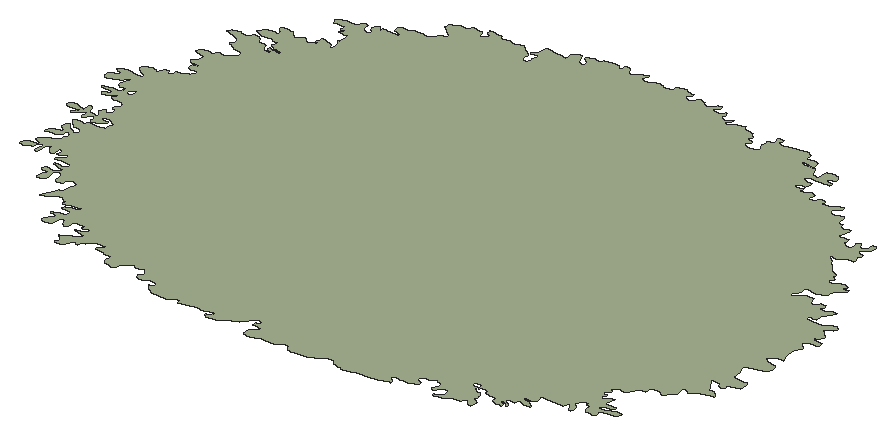
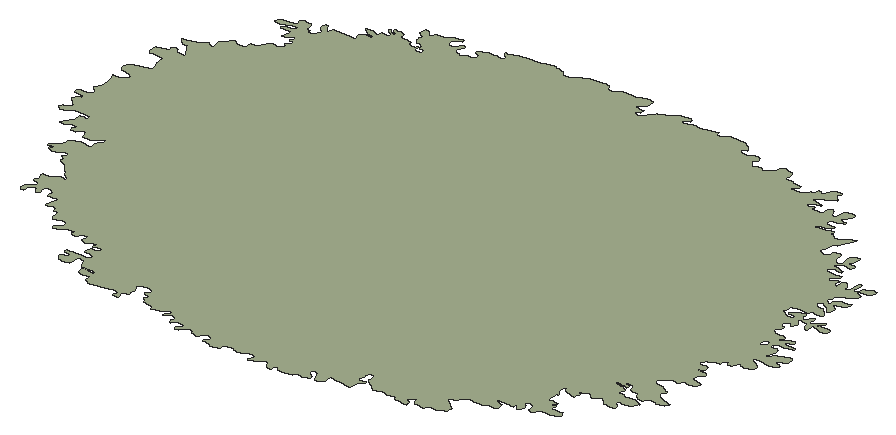
# SketchUp Ruby script. Lengths in inches.
U = 1.inch
M = Sketchup.active_model
def pt(a) = Geom::Point3d.new(a.map { |v| v * U })
def face(e, loops, mat)
  f = e.add_face(loops[0].map { |a| pt(a) })
  loops[1..].each { |l| e.add_face(l.map { |a| pt(a) }).erase! }
  f.material = f.back_material = mat if mat
  f
end
# faces: each face lists its corners as indices into pts; further lists are holes
def faces(e, pts, list, mat = nil) = list.each { |f| face(e, (f[0].is_a?(Array) ? f : [f]).map { |l| l.map { |i| pts[i] } }, mat) }
# xy, xz, yz: faces in a plane at the given z, y or x. An outline is a flat list of corners, or four numbers for a rectangle; further outlines are holes
def ring(l) = l.size == 4 ? [[l[0], l[1]], [l[2], l[1]], [l[2], l[3]], [l[0], l[3]]] : l.each_slice(2).to_a
def flat(e, list, mat, &to3) = list.each { |f| face(e, (f[0].is_a?(Array) ? f : [f]).map { |l| ring(l).map { |u, v| to3.(u, v) } }, mat) }
def xy(e, z, list, mat = nil) = flat(e, list, mat) { |x, y| [x, y, z] }
def xz(e, y, list, mat = nil) = flat(e, list, mat) { |x, z| [x, y, z] }
def yz(e, x, list, mat = nil) = flat(e, list, mat) { |y, z| [x, y, z] }
def lines(e, pts, list) = list.each { |a, b| e.add_line(pt(pts[a]), pt(pts[b])) }
# prism: a flat outline (further loops are holes) pulled along v
def prism(e, loops, v, mat = nil)
  f = face(e, loops, mat); d = Geom::Vector3d.new(v.map { |x| x * U })
  f.pushpull(f.normal.samedirection?(d) ? d.length : -d.length)
end
def box(e, o, s, mat = nil) = prism(e, [[o, [o[0] + s[0], o[1], o[2]], [o[0] + s[0], o[1] + s[1], o[2]], [o[0], o[1] + s[1], o[2]]]], [0, 0, s[2]], mat)
def at(x, y, z, deg = 0) = Geom::Transformation.translation(pt([x, y, z])) * Geom::Transformation.rotation(ORIGIN, Z_AXIS, deg.degrees)
def axes(o, x, y, z) = Geom::Transformation.new([*x, 0, *y, 0, *z, 0, *pt(o).to_a, 1])
def part(name) = M.definitions.add(name)
# library, detail: a bought-in or finely detailed component or shape, given as its bounding box
def library(name, o, s) = part(name).tap { |d| box(d.entities, o, s) }
def detail(e, o, s) = box(e.add_group.entities, o, s)
def put(e, d, t, mat = nil) = e.add_instance(d, t).tap { |i| i.material = mat if mat }
def group(e, t, mat = nil) = e.add_group.tap { |g| g.transformation = t; g.material = mat if mat }.entities
root = M.entities
M.materials.add("Boxwoodplan").color = [166, 177, 144]
xy(root,9.058,[[[229.854,67.129,229.743,67.133,229.648,67.159,229.592,67.215,229.591,67.317,229.617,67.382,229.68,67.445,229.729,67.509,229.788,67.606,229.601,67.635,229.511,67.644,229.531,67.732,229.617,67.79,229.648,67.8,229.643,67.846,229.554,67.877,229.438,67.837,229.341,67.706,229.199,67.551,229.038,67.464,228.932,67.441,228.872,67.416,228.856,67.373,228.711,67.281,228.518,67.251,228.429,67.26,228.348,67.306,228.348,67.328,228.394,67.359,228.484,67.437,228.553,67.483,228.463,67.498,228.351,67.48,228.231,67.436,228.037,67.454,227.94,67.447,227.814,67.403,227.613,67.356,227.524,67.349,227.486,67.443,227.478,67.465,227.411,67.473,227.322,67.454,227.154,67.336,226.954,67.328,226.724,67.353,226.557,67.446,226.415,67.61,226.598,67.702,226.499,67.756,226.363,67.772,226.237,67.749,226.164,67.697,226.084,67.672,225.968,67.738,225.926,67.806,226.013,67.847,226.04,67.907,226.045,67.957,226.004,68.009,225.931,68.085,225.846,68.117,225.759,68.064,225.692,68.038,225.636,68.08,225.62,68.103,225.596,68.121,225.566,68.111,225.487,68.058,225.415,68.01,225.339,67.923,225.328,67.79,225.256,67.749,225.206,67.723,225.146,67.725,225.047,67.746,224.961,67.793,224.917,67.861,224.908,67.951,224.917,68.018,224.93,68.04,224.911,68.08,224.698,68.1,224.766,68.135,224.739,68.136,224.647,68.13,224.477,68.146,224.4,68.173,224.383,68.206,224.397,68.224,224.523,68.314,224.52,68.371,224.436,68.393,224.276,68.39,224.146,68.319,224.048,68.233,223.974,68.199,223.926,68.172,223.925,68.154,223.962,68.101,223.946,68.046,223.875,68.081,223.812,68.121,223.751,68.072,223.728,68.017,223.697,67.904,223.649,67.855,223.576,67.822,223.485,67.816,223.415,67.841,223.397,67.874,223.404,67.892,223.425,67.932,223.447,67.991,223.416,68.048,223.315,68.149,223.429,68.229,223.49,68.269,223.569,68.285,223.637,68.315,223.692,68.37,223.776,68.476,223.705,68.503,223.625,68.511,223.493,68.53,223.454,68.565,223.462,68.584,223.536,68.62,223.698,68.657,223.741,68.709,223.736,68.748,223.71,68.764,223.56,68.711,223.514,68.732,223.515,68.752,223.537,68.814,223.376,68.825,223.296,68.833,223.242,68.826,223.234,68.806,223.218,68.71,223.203,68.642,223.162,68.591,223.115,68.578,223.095,68.594,223.036,68.639,222.992,68.757,222.952,68.783,222.925,68.784,222.872,68.777,222.865,68.757,222.863,68.641,222.808,68.523,222.748,68.449,222.668,68.419,222.589,68.422,222.542,68.448,222.509,68.506,222.51,68.564,222.563,68.677,222.677,68.784,222.698,68.803,222.684,68.823,222.658,68.829,222.577,68.847,222.497,68.86,222.47,68.875,222.476,68.895,222.497,68.914,222.645,68.982,222.807,69.005,222.849,69.108,222.823,69.169,222.776,69.191,222.748,69.187,222.585,69.168,222.545,69.2,222.551,69.22,222.579,69.279,222.736,69.334,222.908,69.403,222.957,69.442,222.943,69.463,222.847,69.436,222.675,69.417,222.531,69.372,222.442,69.386,222.415,69.392,222.422,69.412,222.442,69.426,222.497,69.47,222.47,69.507,222.442,69.503,222.36,69.511,222.305,69.56,222.291,69.601,222.263,69.597,222.181,69.575,222.024,69.489,221.874,69.413,221.8,69.38,221.745,69.392,221.758,69.412,221.778,69.452,221.804,69.469,221.829,69.55,221.878,69.65,221.91,69.759,221.961,69.812,222.035,69.852,222.079,69.972,222.101,70.112,222.12,70.227,222.116,70.285,222.071,70.321,221.991,70.335,221.904,70.335,221.831,70.31,221.821,70.245,221.821,70.184,221.788,70.124,221.7,70.087,221.644,70.096,221.605,70.155,221.595,70.216,221.569,70.337,221.563,70.4,221.523,70.453,221.495,70.475,221.458,70.491,221.399,70.479,221.364,70.46,221.363,70.428,221.355,70.366,221.357,70.229,221.382,70.167,221.374,70.103,221.324,70.038,221.275,70.01,221.237,69.998,221.2,70.003,221.158,70.011,221.14,70.039,221.136,70.166,221.157,70.223,221.202,70.276,221.218,70.306,221.209,70.334,221.152,70.34,221.071,70.346,221.033,70.362,221.01,70.39,221.007,70.453,221.023,70.483,221.057,70.499,221.23,70.472,221.308,70.497,221.358,70.526,221.418,70.573,221.432,70.636,221.409,70.662,221.365,70.664,221.287,70.67,221.195,70.681,221.094,70.717,221.076,70.746,221.081,70.76,221.101,70.763,221.16,70.775,221.336,70.761,221.425,70.787,221.438,70.844,221.412,70.907,221.34,70.946,221.261,70.953,221.147,70.946,221.048,70.921,220.964,70.939,220.96,70.968,220.981,70.997,221.027,71.054,221.094,71.11,221.147,71.19,221.138,71.224,221.094,71.241,221.029,71.24,220.911,71.14,220.871,71.141,220.837,71.161,220.858,71.22,220.875,71.287,220.831,71.35,220.791,71.366,220.771,71.367,220.766,71.352,220.77,71.306,220.767,71.164,220.726,71.102,220.686,71.108,220.652,71.131,220.554,71.262,220.529,71.327,220.505,71.355,220.489,71.344,220.434,71.293,220.399,71.234,220.418,71.103,220.423,71.037,220.403,70.971,220.354,70.962,220.319,70.978,220.309,71.023,220.329,71.155,220.339,71.233,220.339,71.27,220.324,71.282,220.309,71.272,220.229,71.237,220.19,71.183,220.18,71.12,220.141,71.077,220.004,70.987,219.965,70.977,219.92,70.986,219.841,71.026,219.82,71.056,219.824,71.089,219.857,71.151,219.955,71.237,220.044,71.263,220.134,71.263,220.229,71.267,220.169,71.318,220.017,71.404,220.001,71.466,220.054,71.503,220.145,71.573,220.264,71.635,220.383,71.709,220.418,71.723,220.444,71.746,220.471,71.789,220.474,71.882,220.506,72.003,220.507,72.065,220.486,72.086,220.465,72.095,220.402,72.109,220.368,72.104,220.365,72.088,220.376,71.996,220.335,71.934,220.287,71.899,220.209,71.871,220.138,71.858,219.978,71.833,219.943,71.839,219.929,71.853,219.93,71.86,219.938,71.901,219.955,71.947,219.997,71.995,220.067,72.042,220.125,72.063,220.184,72.065,220.222,72.068,220.242,72.075,220.265,72.096,220.261,72.121,220.206,72.151,220.138,72.207,220.106,72.264,220.102,72.331,220.115,72.382,220.168,72.426,220.194,72.432,220.205,72.425,220.224,72.411,220.267,72.35,220.316,72.304,220.445,72.226,220.518,72.192,220.554,72.177,220.574,72.184,220.598,72.206,220.604,72.222,220.616,72.263,220.6,72.32,220.558,72.366,220.525,72.389,220.492,72.401,220.432,72.401,220.358,72.404,220.314,72.446,220.228,72.519,220.17,72.569,220.131,72.617,220.131,72.646,220.155,72.671,220.212,72.698,220.247,72.703,220.288,72.7,220.348,72.679,220.409,72.677,220.445,72.684,220.48,72.726,220.528,72.757,220.588,72.764,220.659,72.764,220.8125,72.771,220.953,72.792,220.985,72.808,220.986,72.826,220.98,72.868,220.969,72.913,220.98,72.957,221.01,73.06,220.996,73.083,220.974,73.097,220.917,73.126,220.863,73.164,220.791,73.192,220.718,73.195,220.667,73.184,220.646,73.17,220.621,73.119,220.626,73.098,220.638,73.093,220.661,73.088,220.812,73.076,220.838,73.071,220.844,73.0625,220.834,73.046,220.795,73.007,220.749,72.964,220.685,72.928,220.623,72.884,220.55,72.849,220.513,72.852,220.494,72.863,220.468,72.9,220.461,72.995,220.444,73.02,220.462,73.034,220.469,73.077,220.463,73.088,220.451,73.088,220.437,73.087,220.411,73.083,220.378,73.076,220.361,73.065,220.28,72.97,220.248,72.915,220.217,72.892,220.194,72.895,220.168,72.916,220.159,72.932,220.153,72.973,220.181,73.057,220.187,73.102,220.178,73.13,220.157,73.137,220.119,73.128,220.099,73.114,220.053,73.064,219.932,72.957,219.895,72.932,219.87,72.927,219.832,72.935,219.82,72.951,219.912,73.057,219.974,73.102,219.988,73.129,219.988,73.145,219.979,73.152,219.967,73.148,219.953,73.143,219.921,73.131,219.838,73.108,219.67,73.089,219.597,73.096,219.55,73.121,219.528,73.149,219.527,73.165,219.544,73.217,219.591,73.264,219.652,73.281,219.722,73.284,219.797,73.266,219.924,73.223,220.01,73.197,220.022,73.201,220.022,73.209,220.021,73.22,220.012,73.239,219.988,73.287,219.986,73.342,219.994,73.407,220.005,73.437,220.023,73.45,220.071,73.413,220.111,73.363,220.138,73.317,220.147,73.255,220.16,73.204,220.174,73.176,220.198,73.175,220.332,73.157,220.405,73.144,220.44,73.14,220.458,73.154,220.474,73.202,220.418,73.244,220.36,73.309,220.342,73.335,220.342,73.352,220.376,73.46,220.406,73.483,220.434,73.489,220.448,73.477,220.457,73.459,220.486,73.414,220.498,73.39,220.51,73.391,220.531,73.404,220.611,73.482,220.627,73.528,220.629,73.579,220.615,73.611,220.594,73.623,220.53,73.646,220.491,73.666,220.482,73.687,220.498,73.736,220.554,73.773,220.589,73.795,220.602,73.816,220.609,73.869,220.608,73.916,220.512,73.992,220.369,74.014,220.306,74.031,220.272,74.013,220.243,74.014,220.174,74.031,220.155,74.058,220.165,74.082,220.291,74.185,220.284,74.217,220.262,74.233,220.218,74.225,220.189,74.216,220.063,74.154,220.023,74.107,219.973,74.063,219.904,74.049,219.876,74.05,219.829,74.102,219.857,74.126,219.875,74.165,219.907,74.188,220,74.22,220.045,74.25,220.035,74.281,220.022,74.283,220.012,74.276,219.986,74.27,219.946,74.273,219.811,74.284,219.665,74.3125,219.641,74.327,219.646,74.347,219.671,74.375,219.884,74.435,219.948,74.434,220.008,74.419,220.069,74.391,220.095,74.393,220.102,74.403,220.151,74.48,220.174,74.495,220.181,74.515,220.18,74.557,220.18,74.583,220.17,74.593,220.156,74.591,220.099,74.591,220.041,74.585,219.994,74.568,219.97,74.576,219.95,74.596,219.925,74.63,219.905,74.718,219.915,74.806,219.945,74.848,219.951,74.88,219.964,74.923,220.002,74.944,219.997,74.99,219.975,75.026,219.886,75.003,219.869,74.969,219.87,74.95,219.873,74.886,219.792,74.839,219.651,74.745,219.496,74.7,219.412,74.725,219.37,74.778,219.36,74.904,219.489,74.99,219.571,75.003,219.615,75.027,219.639,75.061,219.637,75.081,219.552,75.112,219.479,75.138,219.417,75.194,219.452,75.249,219.528,75.278,219.624,75.312,219.689,75.311,219.867,75.267,219.96,75.246,220.044,75.25,220.095,75.269,220.101,75.289,220.086,75.355,220.025,75.407,219.98,75.415,219.868,75.485,219.821,75.527,219.806,75.564,219.8,75.617,219.8,75.644,219.8125,75.659,219.855,75.695,219.906,75.709,220.02,75.741,220.05,75.751,220.091,75.75,220.141,75.746,220.153,75.733,220.168,75.703,220.183,75.689,220.192,75.689,220.221,75.692,220.237,75.704,220.257,75.754,220.285,75.787,220.302,75.81,220.304,75.835,220.321,75.86,220.34,75.872,220.388,75.884,220.427,75.877,220.449,75.833,220.453,75.781,220.469,75.755,220.491,75.754,220.532,75.796,220.557,75.838,220.572,75.942,220.587,75.968,220.62,75.975,220.651,75.974,220.671,75.963,220.692,75.94,220.724,75.94,220.776,75.961,220.821,76.007,220.835,76.032,220.824,76.046,220.884,76.043,220.913,76.046,220.928,76.066,220.933,76.114,220.967,76.155,221.002,76.2,220.948,76.243,220.88,76.272,220.843,76.271,220.811,76.261,220.768,76.249,220.727,76.255,220.705,76.271,220.683,76.295,220.66,76.397,220.673,76.423,220.679,76.439,220.689,76.443,220.793,76.463,220.839,76.472,220.858,76.483,220.848,76.486,220.762,76.514,220.696,76.526,220.668,76.519,220.632,76.52,220.596,76.52,220.561,76.532,220.522,76.582,220.504,76.611,220.504,76.642,220.52,76.663,220.549,76.678,220.58,76.697,220.588,76.725,220.618,76.782,220.645,76.836,220.651,76.89,220.643,76.917,220.603,76.928,220.525,76.954,220.352,77.001,220.317,77.018,220.3,77.042,220.335,77.097,220.38,77.131,220.425,77.159,220.48,77.178,220.533,77.1875,220.585,77.184,220.64,77.16,220.696,77.162,220.722,77.167,220.736,77.187,220.753,77.228,220.79,77.264,220.81,77.282,220.837,77.284,220.906,77.267,220.968,77.256,220.994,77.253,221.018,77.268,221.104,77.336,221.192,77.401,221.245,77.498,221.242,77.542,221.2,77.579,221.083,77.617,220.958,77.647,220.871,77.719,220.814,77.755,220.745,77.776,220.717,77.788,220.704,77.808,220.726,77.855,220.774,77.896,220.772,77.981,220.722,78.06,220.592,78.116,220.352,78.196,220.303,78.212,220.283,78.246,220.354,78.31,220.475,78.362,220.581,78.367,220.638,78.353,220.682,78.327,220.73,78.317,220.783,78.326,220.844,78.337,220.874,78.368,220.888,78.448,220.906,78.483,220.959,78.482,221.016,78.471,221.064,78.451,221.131,78.392,221.156,78.358,221.17,78.318,221.171,78.249,221.177,78.245,221.185,78.249,221.212,78.262,221.264,78.268,221.352,78.271,221.432,78.235,221.467,78.17,221.491,78.092,221.561,78.047,221.602,78.035,221.619,78.034,221.646,78.043,221.742,78.05,221.758,78.055,221.738,78.071,221.675,78.095,221.624,78.099,221.585,78.118,221.566,78.152,221.563,78.164,221.567,78.184,221.582,78.191,221.616,78.192,221.658,78.185,221.765,78.156,221.879,78.152,221.931,78.159,221.95,78.162,221.976,78.173,221.932,78.203,221.89,78.213,221.804,78.228,221.746,78.242,221.706,78.244,221.683,78.248,221.658,78.263,221.607,78.289,221.56,78.315,221.537,78.348,221.548,78.404,221.576,78.442,221.617,78.471,221.577,78.502,221.522,78.517,221.48,78.52,221.424,78.528,221.393,78.555,221.376,78.591,221.361,78.6,221.333,78.599,221.217,78.571,221.165,78.557,221.115,78.559,221.068,78.562,221.018,78.578,220.97,78.595,220.93,78.602,220.844,78.65,220.87,78.662,220.871,78.669,220.883,78.709,220.898,78.745,220.924,78.782,220.955,78.814,220.999,78.839,221.052,78.862,221.098,78.873,221.204,78.867,221.281,78.862,221.314,78.858,221.324,78.857,221.324,78.87,221.316,78.912,221.295,78.956,221.259,78.995,221.217,79.026,221.184,79.073,221.186,79.096,221.196,79.117,221.244,79.147,221.296,79.17,221.322,79.169,221.348,79.163,221.403,79.148,221.47,79.142,221.518,79.127,221.541,79.114,221.56,79.095,221.603,79.055,221.642,79.02,221.687,78.989,221.744,78.976,221.797,78.981,221.843,79.01,221.874,79.046,221.923,79.084,221.949,79.083,221.972,79.069,222.012,79.027,222.059,78.994,222.1875,79.019,222.262,79.037,222.303,79.065,222.309,79.085,222.287,79.102,222.236,79.124,222.227,79.147,222.235,79.169,222.25,79.214,222.257,79.273,222.261,79.299,222.284,79.315,222.312,79.316,222.342,79.308,222.384,79.288,222.518,79.248,222.578,79.226,222.618,79.193,222.644,79.153,222.659,79.13,222.666,79.123,222.676,79.126,222.684,79.131,222.716,79.176,222.722,79.212,222.712,79.315,222.691,79.362,222.667,79.397,222.631,79.436,222.621,79.466,222.633,79.477,222.644,79.475,222.665,79.476,222.665,79.484,222.67,79.508,222.662,79.549,222.648,79.705,222.65,79.782,222.534,79.802,222.437,79.804,222.375,79.8125,222.357,79.819,222.343,79.83,222.356,79.839,222.469,79.882,222.503,79.911,222.503,79.924,222.48,79.948,222.444,79.952,222.391,79.94,222.343,79.918,222.325,79.919,222.31,79.945,222.337,80.028,222.339,80.069,222.339,80.082,222.315,80.103,222.226,80.085,222.113,80.088,222.003,80.105,221.942,80.185,221.94,80.213,221.978,80.25,222.075,80.303,222.123,80.33,222.178,80.335,222.302,80.332,222.394,80.337,222.453,80.346,222.493,80.384,222.534,80.418,222.541,80.461,222.568,80.5,222.623,80.513,222.661,80.509,222.704,80.475,222.715,80.389,222.722,80.3,222.745,80.257,222.801,80.231,222.892,80.212,222.947,80.234,222.965,80.276,222.942,80.319,222.896,80.355,222.839,80.442,222.875,80.521,222.95,80.603,222.969,80.606,222.992,80.576,223.011,80.528,223.086,80.447,223.113,80.421,223.104,80.475,223.086,80.57,223.143,80.587,223.204,80.582,223.331,80.578,223.444,80.575,223.565,80.557,223.584,80.557,223.571,80.587,223.521,80.629,223.39,80.681,223.352,80.689,223.33,80.735,223.332,80.826,223.366,80.871,223.415,80.896,223.531,80.901,223.628,80.91,223.723,80.977,223.85,80.982,223.966,80.971,224.061,80.953,224.182,80.946,224.225,80.991,224.239,81.038,224.282,81.133,224.371,81.187,224.491,81.244,224.502,81.26,224.486,81.294,224.445,81.332,224.338,81.413,224.269,81.487,224.212,81.528,224.155,81.57,224.185,81.577,224.184,81.591,224.18,81.612,224.168,81.679,224.172,81.709,224.207,81.744,224.289,81.785,224.372,81.821,224.411,81.827,224.467,81.826,224.553,81.816,224.577,81.808,224.601,81.81,224.632,81.843,224.684,81.918,224.72,81.932,224.777,81.936,224.879,81.93,224.975,81.898,225.008,81.877,225.037,81.835,225.038,81.765,225.04,81.736,225.045,81.715,225.069,81.704,225.122,81.715,225.167,81.745,225.228,81.798,225.253,81.822,225.275,81.834,225.287,81.85,225.203,81.897,225.165,81.913,225.121,81.956,225.096,82.036,225.097,82.067,225.156,82.083,225.347,82.055,225.444,82.039,225.48,82.026,225.479,81.98,225.489,81.952,225.55,81.948,225.654,81.962,225.755,81.975,225.798,81.971,225.844,81.957,225.872,81.934,225.896,81.933,225.921,81.943,226.065,81.972,226.106,81.981,226.159,81.987,226.195,81.984,226.239,81.957,226.27,81.886,226.296,81.863,226.341,81.844,226.381,81.833,226.421,81.808,226.473,81.753,226.526,81.696,226.513,81.619,226.507,81.545,226.521,81.515,226.552,81.485,226.578,81.461,226.625,81.453,226.662,81.45,226.706,81.481,226.72,81.512,226.721,81.553,226.709,81.628,226.745,81.787,226.734,81.817,226.716,81.829,226.693,81.833,226.654,81.834,226.602,81.828,226.565,81.826,226.519,81.835,226.493,81.858,226.501,81.88,226.528,81.896,226.568,81.91,226.613,81.937,226.638,82.013,226.641,82.178,226.642,82.21,226.664,82.228,226.691,82.233,226.789,82.222,226.988,82.201,227.08,82.19,227.168,82.169,227.255,82.153,227.306,82.147,227.302,82.355,227.37,82.427,227.454,82.486,227.509,82.477,227.536,82.441,227.585,82.37,227.608,82.297,227.616,82.26,227.614,82.241,227.641,82.206,227.746,82.173,227.798,82.173,227.836,82.204,227.839,82.279,227.737,82.36,227.659,82.419,227.671,82.453,227.715,82.49,227.808,82.541,227.858,82.55,227.939,82.538,228.044,82.537,228.066,82.615,228.276,82.643,228.377,82.661,228.484,82.647,228.564,82.578,228.597,82.543,228.623,82.541,228.663,82.568,228.661,82.643,228.653,82.685,228.665,82.72,228.716,82.729,228.771,82.715,228.842,82.621,228.863,82.548,228.896,82.513,228.944,82.498,228.995,82.503,229.042,82.53,229.13,82.613,229.211,82.668,229.3125,82.715,229.361,82.7,229.374,82.663,229.323,82.592,229.297,82.557,229.305,82.515,229.393,82.457,229.493,82.443,229.544,82.452,229.593,82.498,229.672,82.566,229.786,82.581,229.901,82.553,229.933,82.523,230.009,82.492,230.11,82.511,230.191,82.565,230.191,82.678,230.249,82.721,230.362,82.745,230.467,82.74,230.548,82.681,230.694,82.66,230.747,82.651,230.753,82.614,230.68,82.546,230.647,82.473,230.659,82.437,230.73,82.396,230.833,82.401,230.885,82.433,230.905,82.472,230.926,82.544,230.974,82.567,230.998,82.579,231.05,82.579,231.153,82.541,231.196,82.47,231.281,82.417,231.412,82.447,231.446,82.478,231.453,82.52,231.492,82.603,231.599,82.622,231.629,82.592,231.635,82.55,231.583,82.466,231.534,82.448,231.507,82.413,231.568,82.349,231.698,82.337,231.789,82.373,231.857,82.444,231.881,82.45,231.89,82.433,231.909,82.392,231.933,82.357,231.921,82.301,231.902,82.257,231.92,82.222,232.009,82.179,232.117,82.184,232.172,82.203,232.222,82.258,232.239,82.273,232.242,82.255,232.228,82.212,232.156,82.132,232.122,82.102,232.133,82.066,232.18,82.047,232.237,82.048,232.334,82.088,232.416,82.146,232.636,82.225,232.657,82.153,232.68,82.123,232.732,82.118,232.847,82.11,232.971,82.084,232.986,82.013,233.009,81.983,233.056,81.964,233.079,81.93,233.064,81.892,233.038,81.795,233.154,81.773,233.2,81.755,233.211,81.72,233.137,81.65,233.122,81.613,233.139,81.579,233.214,81.527,233.318,81.5,233.419,81.496,233.531,81.563,233.573,81.639,233.515,81.71,233.482,81.779,233.502,81.885,233.511,81.922,233.482,81.956,233.478,81.992,233.519,82.018,233.62,82.022,233.609,82.122,233.568,82.274,233.617,82.287,233.682,82.275,233.735,82.256,233.767,82.199,233.717,82.131,233.72,82.095,233.767,82.076,233.875,82.076,234.004,82.111,234.512,82.178,234.557,82.168,234.603,82.145,234.65,82.121,234.684,82.097,234.715,82.027,234.697,81.935,234.902,81.949,234.967,81.943,235.051,81.911,235.088,81.805,235.074,81.757,235.057,81.724,235.016,81.717,234.847,81.749,234.782,81.755,234.74,81.755,234.719,81.749,234.716,81.733,234.745,81.685,234.785,81.666,234.833,81.666,235.005,81.681,235.074,81.683,235.159,81.648,235.196,81.609,235.226,81.546,235.294,81.437,235.374,81.398,235.458,81.394,235.489,81.435,235.483,81.518,235.465,81.571,235.472,81.637,235.513,81.687,235.615,81.719,235.724,81.732,235.8125,81.701,235.86,81.659,235.894,81.597,235.895,81.551,235.834,81.495,235.767,81.482,235.726,81.471,235.694,81.437,235.698,81.407,235.748,81.389,235.846,81.363,235.917,81.339,235.937,81.306,235.925,81.275,235.871,81.247,235.783,81.24,235.622,81.233,235.534,81.222,235.446,81.256,235.381,81.269,235.3,81.251,235.243,81.208,235.242,81.143,235.3,81.103,235.387,81.081,235.472,81.066,235.519,81.066,235.553,81.046,235.575,81.003,235.558,80.938,235.523,80.89,235.495,80.866,235.45,80.854,235.307,80.834,235.287,80.829,235.278,80.784,235.283,80.751,235.327,80.732,235.395,80.731,235.436,80.731,235.486,80.746,235.549,80.778,235.563,80.712,235.533,80.665,235.527,80.635,235.566,80.617,235.627,80.622,235.708,80.67,235.764,80.711,235.792,80.736,235.83,80.721,235.894,80.704,235.963,80.651,235.959,80.603,235.916,80.537,235.883,80.472,235.902,80.448,235.949,80.445,236.024,80.456,236.106,80.495,236.145,80.554,236.217,80.597,236.277,80.609,236.314,80.601,236.333,80.577,236.336,80.548,236.319,80.521,236.291,80.497,236.293,80.483,236.313,80.481,236.485,80.499,236.566,80.51,236.633,80.552,236.675,80.589,236.754,80.614,236.851,80.619,236.875,80.595,236.878,80.566,236.717,80.349,236.732,80.304,236.789,80.251,236.872,80.237,236.962,80.255,237.03,80.283,237.114,80.305,237.179,80.213,237.216,79.999,237.217,79.985,237.254,79.974,237.337,79.996,237.348,79.918,237.372,79.871,237.448,79.861,237.586,79.896,237.654,79.893,237.668,79.839,237.6,79.619,237.59,79.567,237.613,79.514,237.679,79.486,237.747,79.496,237.883,79.523,237.903,79.419,237.898,79.316,238.02,79.247,238.152,79.216,238.183,79.318,238.172,79.421,238.15,79.474,238.178,79.525,238.246,79.535,238.285,79.482,238.307,79.429,238.355,79.395,238.433,79.418,238.486,79.467,238.511,79.583,238.514,79.636,238.575,79.659,238.633,79.631,238.663,79.577,238.637,79.455,238.522,79.375,238.469,79.339,238.449,79.282,238.429,79.231,238.451,79.186,238.583,79.161,238.64,79.134,238.644,79.083,238.572,78.997,238.606,78.895,238.636,78.844,238.624,78.794,238.49,78.768,238.388,78.729,238.285,78.658,238.233,78.623,238.168,78.626,238.104,78.659,238.071,78.667,238.045,78.643,238.09,78.549,238.209,78.483,238.255,78.445,238.252,78.396,238.337,78.32,238.504,78.132,238.635,78.05,238.699,78.035,238.736,77.992,238.721,77.898,238.836,77.834,238.773,77.749,238.753,77.697,238.752,77.673,238.783,77.661,238.92,77.679,239.055,77.755,239.184,77.768,239.309,77.734,239.313,77.687,239.246,77.66,239.221,77.644,239.235,77.62,239.3125,77.599,239.384,77.596,239.416,77.595,239.43,77.571,239.341,77.482,239.175,77.322,239.151,77.232,239.147,77.187,239.12,77.142,239.026,77.067,238.898,77.038,238.773,77.043,238.665,77.082,238.595,77.076,238.568,77.004,238.596,76.894,238.566,76.787,238.448,76.72,238.476,76.62,238.614,76.642,238.786,76.833,239.014,76.815,239.09,76.605,239.135,76.595,239.216,76.618,239.304,76.723,239.442,76.735,239.479,76.635,239.429,76.574,239.415,76.539,239.491,76.501,239.63,76.531,239.75,76.598,239.797,76.614,239.886,76.592,239.864,76.477,239.754,76.384,239.689,76.289,239.696,76.113,239.682,76.078,239.59,76.056,239.457,76.087,239.482,75.981,239.614,75.941,239.76,75.936,239.908,75.965,240.145,76.087,240.282,76.099,240.374,76.008,240.341,75.905,240.201,75.849,240.153,75.825,240.125,75.766,240.228,75.675,240.379,75.515,240.347,75.414,240.23,75.359,240.194,75.335,240.233,75.274,240.376,75.269,240.507,75.247,240.518,75.145,240.446,75.089,240.312,75.078,240.187,75.041,240.144,74.942,240.3125,74.761,240.205,74.568,240.209,74.388,240.263,74.176,240.307,74.078,240.174,74.051,240.051,74.008,239.958,73.931,239.93,73.869,240.042,73.801,240.293,73.744,240.37,73.662,240.391,73.559,240.349,73.467,240.235,73.394,239.774,73.234,239.775,73.141,239.819,73.048,239.873,72.954,239.875,72.863,239.866,72.773,239.892,72.719,240.013,72.676,240.138,72.672,240.265,72.682,240.306,72.68,240.364,72.633,240.375,72.453,240.348,72.395,240.239,72.347,240.113,72.33,240.072,72.331,240.025,72.281,240.068,72.191,240.054,72.163,239.97,72.144,239.929,72.145,239.859,72.17,239.826,72.26,239.757,72.292,239.633,72.297,239.591,72.291,239.576,72.233,239.651,72.156,239.738,71.992,239.767,71.969,239.793,71.918,239.81,71.888,239.891,71.877,239.972,71.86,240.057,71.792,240.12,71.71,240.117,71.681,240.032,71.656,239.784,71.616,239.588,71.488,239.515,71.469,239.421,71.544,239.381,71.553,239.317,71.52,239.32,71.435,239.376,71.27,239.334,71.264,239.3,71.219,239.251,71.18,239.198,71.066,239.159,71.019,239.124,71,239.089,71.013,238.966,71.1,238.904,71.115,238.861,71.116,238.816,71.098,238.753,71.063,238.723,70.991,238.732,70.938,238.714,70.874,238.553,70.852,238.5,70.81,238.468,70.759,238.422,70.718,238.41,70.655,238.379,70.609,238.345,70.583,238.307,70.573,238.238,70.564,238.14,70.575,238.08,70.55,238.019,70.502,237.989,70.457,238.063,70.419,238.09,70.376,238.054,70.32,238,70.284,237.979,70.225,237.978,70.209,237.976,70.194,237.996,70.186,238.067,70.18,238.093,70.182,238.113,70.182,238.117,70.166,238.08,70.097,238.06,70.049,238.057,70.02,238.098,70.018,238.238,70.094,238.306,70.11,238.388,70.107,238.371,70.004,238.354,69.89,238.354,69.843,238.377,69.82,238.417,69.818,238.48,69.845,238.561,69.846,238.62,69.832,238.66,69.827,238.667,69.798,238.627,69.76,238.548,69.73,238.481,69.722,238.398,69.696,238.359,69.658,238.343,69.602,238.346,69.587,238.386,69.586,238.469,69.611,238.626,69.673,238.781,69.703,238.906,69.705,238.959,69.685,238.934,69.611,238.913,69.569,238.851,69.518,238.699,69.492,238.559,69.491,238.499,69.482,238.468,69.427,238.493,69.308,238.478,69.264,238.397,69.243,238.261,69.255,238.203,69.261,238.159,69.314,238.151,69.426,238.15,69.468,238.138,69.496,238.13,69.511,238.11,69.512,238.051,69.525,238.047,69.581,238.048,69.595,238.045,69.61,238.025,69.614,237.946,69.617,237.888,69.591,237.844,69.536,237.806,69.499,237.782,69.44,237.792,69.391,237.848,69.354,237.923,69.254,237.919,69.155,237.911,69.115,237.903,69.088,237.872,69.066,237.853,69.067,237.831,69.098,237.802,69.157,237.737,69.258,237.696,69.298,237.683,69.312,237.672,69.299,237.665,69.271,237.662,69.227,237.643,69.173,237.637,69.16,237.607,69.144,237.523,69.137,237.383,69.139,237.096,69.14,237.039,69.162,236.952,69.173,236.932,69.163,236.926,69.133,236.977,69.074,237.002,68.976,236.995,68.936,236.964,68.896,236.939,68.889,236.879,68.88,236.776,68.88,236.679,68.884,236.63,68.853,236.686,68.829,236.787,68.814,236.894,68.78,236.969,68.726,237.05,68.654,237.032,68.629,236.972,68.614,236.871,68.621,236.833,68.63,236.783,68.65,236.734,68.684,236.684,68.708,236.649,68.63,236.64,68.558,236.599,68.545,236.543,68.558,236.499,68.589,236.486,68.6,236.467,68.608,236.456,68.59,236.422,68.513,236.423,68.485,236.457,68.448,236.549,68.416,236.587,68.383,236.601,68.34,236.599,68.326,236.579,68.323,236.537,68.36,236.457,68.409,236.363,68.427,236.306,68.429,236.295,68.415,236.316,68.39,236.43,68.347,236.466,68.335,236.49,68.292,236.486,68.264,236.484,68.251,236.441,68.249,236.329,68.26,236.224,68.295,236.189,68.325,236.18,68.371,236.178,68.441,236.128,68.461,236.068,68.442,235.968,68.449,235.87,68.467,235.843,68.489,235.818,68.526,235.822,68.568,235.828,68.583,235.79,68.591,235.696,68.616,235.657,68.618,235.638,68.619,235.603,68.606,235.591,68.577,235.572,68.571,235.545,68.597,235.541,68.612,235.572,68.635,235.587,68.646,235.58,68.671,235.492,68.729,235.455,68.752,235.436,68.756,235.356,68.716,235.336,68.71,235.324,68.681,235.347,68.59,235.443,68.587,235.481,68.582,235.512,68.541,235.505,68.513,235.499,68.499,235.506,68.471,235.618,68.434,235.705,68.396,235.767,68.338,235.783,68.3125,235.782,68.299,235.748,68.283,235.728,68.273,235.759,68.251,235.813,68.225,235.825,68.2,235.775,68.168,235.763,68.141,235.788,68.106,235.873,68.062,235.95,67.994,235.95,67.851,235.928,67.825,235.876,67.814,235.822,67.829,235.785,67.874,235.744,67.939,235.727,67.949,235.689,67.944,235.636,67.926,235.615,67.897,235.616,67.854,235.615,67.84,235.581,67.828,235.405,67.819,235.396,67.826,235.349,67.808,235.305,67.777,235.221,67.692,235.168,67.661,235.095,67.651,234.957,67.643,234.903,67.658,234.9,67.698,235.009,67.762,235.11,67.834,235.107,67.937,235.1,67.98,235.101,67.994,235.069,68.015,235.01,68.034,234.935,68.034,234.852,67.95,234.832,67.911,234.774,67.866,234.76,67.857,234.723,67.865,234.687,67.88,234.674,67.907,234.715,67.999,234.774,68.094,234.776,68.135,234.708,68.189,234.596,68.224,234.545,68.246,234.507,68.238,234.483,68.215,234.449,68.171,234.416,68.156,234.374,68.157,234.318,68.166,234.28,68.168,234.242,68.145,234.162,68.05,234.175,68.01,234.249,67.97,234.304,67.938,234.332,67.917,234.341,67.89,234.317,67.851,234.256,67.807,234.155,67.756,234.099,67.735,234.026,67.738,233.971,67.76,233.898,67.769,233.852,67.745,233.816,67.743,233.784,67.76,233.729,67.766,233.656,67.752,233.633,67.717,233.644,67.659,233.74,67.575,233.768,67.536,233.768,67.497,233.75,67.492,233.461,67.391,233.185,67.369,232.952,67.373,232.862,67.371,232.739,67.31,232.636,67.275,232.539,67.279,232.502,67.281,232.452,67.299,232.404,67.328,232.344,67.325,232.255,67.334,232.171,67.376,232.111,67.433,232.079,67.478,232.021,67.491,231.921,67.479,231.826,67.438,231.745,67.398,231.646,67.325,231.549,67.269,231.456,67.24,231.215,67.222,231.025,67.186,230.929,67.19,230.864,67.284,230.833,67.351,230.744,67.365,230.653,67.352,230.557,67.28,230.492,67.217,230.402,67.21,230.226,67.233,230.04,67.24,229.962,67.189],[220.362,74.415,220.405,74.419,220.424,74.422,220.45,74.431,220.462,74.474,220.463,74.513,220.47,74.597,220.462,74.631,220.45,74.643,220.451,74.658,220.407,74.635,220.351,74.612,220.332,74.606,220.316,74.59,220.294,74.557,220.285,74.52,220.287,74.476,220.306,74.437,220.324,74.421]]],"Boxwoodplan")
